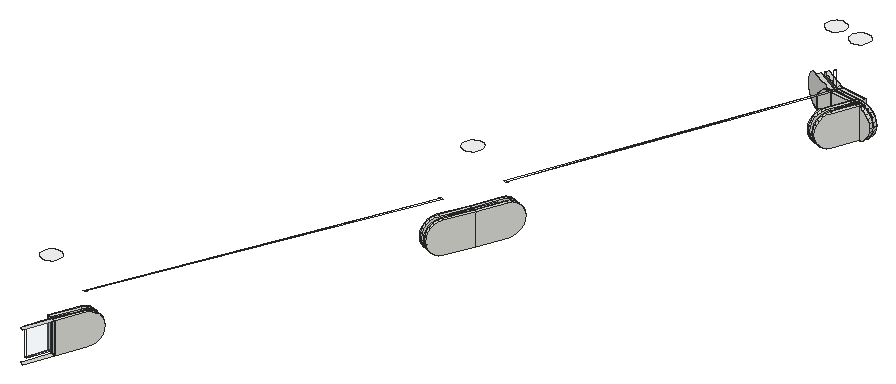
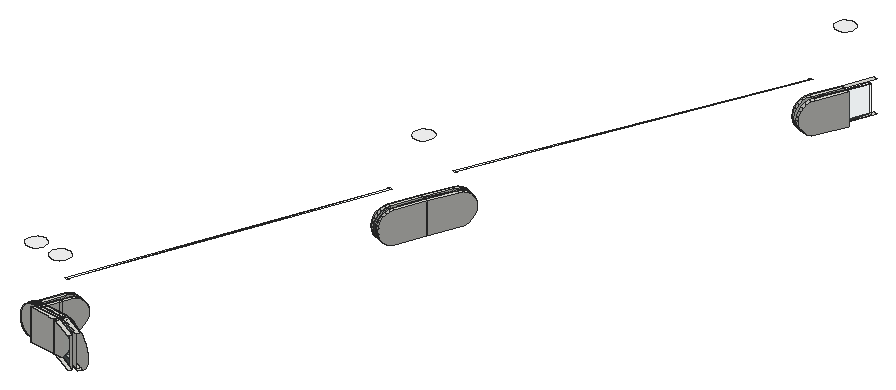
# SketchUp Ruby script. Lengths in inches.
U = 1.inch
M = Sketchup.active_model
def pt(a) = Geom::Point3d.new(a.map { |v| v * U })
def face(e, loops, mat)
  f = e.add_face(loops[0].map { |a| pt(a) })
  loops[1..].each { |l| e.add_face(l.map { |a| pt(a) }).erase! }
  f.material = f.back_material = mat if mat
  f
end
# faces: each face lists its corners as indices into pts; further lists are holes
def faces(e, pts, list, mat = nil) = list.each { |f| face(e, (f[0].is_a?(Array) ? f : [f]).map { |l| l.map { |i| pts[i] } }, mat) }
# xy, xz, yz: faces in a plane at the given z, y or x. An outline is a flat list of corners, or four numbers for a rectangle; further outlines are holes
def ring(l) = l.size == 4 ? [[l[0], l[1]], [l[2], l[1]], [l[2], l[3]], [l[0], l[3]]] : l.each_slice(2).to_a
def flat(e, list, mat, &to3) = list.each { |f| face(e, (f[0].is_a?(Array) ? f : [f]).map { |l| ring(l).map { |u, v| to3.(u, v) } }, mat) }
def xy(e, z, list, mat = nil) = flat(e, list, mat) { |x, y| [x, y, z] }
def xz(e, y, list, mat = nil) = flat(e, list, mat) { |x, z| [x, y, z] }
def yz(e, x, list, mat = nil) = flat(e, list, mat) { |y, z| [x, y, z] }
def lines(e, pts, list) = list.each { |a, b| e.add_line(pt(pts[a]), pt(pts[b])) }
# prism: a flat outline (further loops are holes) pulled along v
def prism(e, loops, v, mat = nil)
  f = face(e, loops, mat); d = Geom::Vector3d.new(v.map { |x| x * U })
  f.pushpull(f.normal.samedirection?(d) ? d.length : -d.length)
end
def box(e, o, s, mat = nil) = prism(e, [[o, [o[0] + s[0], o[1], o[2]], [o[0] + s[0], o[1] + s[1], o[2]], [o[0], o[1] + s[1], o[2]]]], [0, 0, s[2]], mat)
def at(x, y, z, deg = 0) = Geom::Transformation.translation(pt([x, y, z])) * Geom::Transformation.rotation(ORIGIN, Z_AXIS, deg.degrees)
def axes(o, x, y, z) = Geom::Transformation.new([*x, 0, *y, 0, *z, 0, *pt(o).to_a, 1])
def part(name) = M.definitions.add(name)
# library, detail: a bought-in or finely detailed component or shape, given as its bounding box
def library(name, o, s) = part(name).tap { |d| box(d.entities, o, s) }
def detail(e, o, s) = box(e.add_group.entities, o, s)
def put(e, d, t, mat = nil) = e.add_instance(d, t).tap { |i| i.material = mat if mat }
def group(e, t, mat = nil) = e.add_group.tap { |g| g.transformation = t; g.material = mat if mat }.entities
root = M.entities
M.materials.add("Glass_Safety_01").color = [204, 235, 244]
M.materials["Glass_Safety_01"].alpha = 0.1
M.materials.add("[Color_000]").color = [255, 255, 255]
xy(root,351.283,[[963.05,809.92,962.794,810.021,962.855,810.177,963.512,811.85,963.765,811.74],[963.765,811.74,963.512,811.85,963.513,811.853,963.77,811.753,963.767,811.746],[963.77,811.753,963.513,811.853,964.298,813.655,964.551,813.545],[963.332,811.929,963.079,812.039,963.865,813.843,964.118,813.733],[973.145,833.277,972.892,833.387,972.953,833.526,973.678,835.192,973.931,835.082],
  [972.711,833.465,972.459,833.576,973.241,835.37,973.496,835.268,972.772,833.605],[973.935,835.091,973.679,835.194,974.413,837.021,974.669,836.918],[973.496,835.268,973.241,835.37,973.245,835.38,973.497,835.27],[973.497,835.27,973.245,835.38,973.975,837.197,974.231,837.094],[982.068,855.317,981.812,855.42,981.873,855.571,982.412,856.912,982.491,856.9,982.519,857.095,982.531,857.173,982.539,857.227,982.546,857.247,982.802,857.144],
  [981.629,855.494,981.374,855.596,981.931,856.982,982.211,856.941,981.69,855.645],[982.491,856.9,982.412,856.912,982.487,857.1,982.519,857.095],[982.412,856.912,982.401,856.913,982.43,857.108,982.487,857.1],[982.401,856.913,982.211,856.941,982.287,857.129,982.43,857.108],[982.211,856.941,981.931,856.982,982.006,857.17,982.287,857.129],
  [981.931,856.982,980.543,857.184,980.572,857.379,982.006,857.17],[982.519,857.095,982.487,857.1,982.518,857.175,982.531,857.173],[982.487,857.1,982.43,857.108,982.441,857.186,982.518,857.175],[982.43,857.108,982.287,857.129,982.317,857.204,982.441,857.186],[982.287,857.129,982.006,857.17,982.037,857.245,982.317,857.204],
  [982.006,857.17,980.572,857.379,980.583,857.457,982.037,857.245],[982.531,857.173,982.518,857.175,982.539,857.227],[982.518,857.175,982.441,857.186,982.317,857.204,982.364,857.32,982.108,857.423,982.037,857.245,980.583,857.457,980.611,857.652,980.63,857.649,980.646,857.64,980.649,857.646,982.469,857.381,982.559,857.368,982.539,857.227],[980.543,857.184,980.453,857.197,980.474,857.338,980.545,857.462,980.583,857.457,980.572,857.379],[982.317,857.204,982.037,857.245,982.108,857.423,982.364,857.32],
  [980.412,857.229,978.702,858.205,978.839,858.444,980.548,857.469,980.545,857.462,980.493,857.47,980.474,857.338],[980.474,857.338,980.493,857.47,980.545,857.462],[982.469,857.381,980.649,857.646,980.782,857.879,980.721,857.914,982.509,857.653],[980.646,857.64,980.63,857.649,980.649,857.646],[980.649,857.646,980.63,857.649,980.528,857.707,980.561,857.9375,980.721,857.914,980.782,857.879],
  [980.63,857.649,980.611,857.652,980.521,857.665,980.528,857.707],[980.528,857.707,978.936,858.615,979.073,858.855,980.721,857.914,980.561,857.9375]])
xy(root,351.362,[[962.9375,810.388,962.754,810.46,963.33,811.925,963.422,811.889,963.512,811.85],[963.512,811.85,963.422,811.889,963.513,811.853,963.513,811.852],[963.513,811.853,963.422,811.889,963.332,811.929,963.96,813.372,964.141,813.294],[973.049,833.748,972.869,833.826,973.496,835.268,973.588,835.231,973.678,835.192],[973.679,835.194,973.588,835.231,973.497,835.27,974.084,836.729,974.267,836.655],
  [973.588,835.231,973.496,835.268,973.497,835.269,973.497,835.27],[981.959,855.785,981.776,855.859,982.317,857.204,982.441,857.186,982.455,857.283,982.546,857.247],[982.441,857.186,982.317,857.204,982.364,857.32,982.455,857.283],[982.317,857.204,982.141,857.23,982.17,857.424,982.469,857.381,982.455,857.283,982.364,857.32],[982.141,857.23,980.883,857.413,980.911,857.608,982.17,857.424],
  [980.883,857.413,980.583,857.457,980.597,857.554,980.646,857.64,980.63,857.649,980.911,857.608],[980.548,857.469,979.181,858.249,979.278,858.42,980.63,857.649,980.611,857.652,980.597,857.554],[980.597,857.554,980.611,857.652,980.63,857.649,980.646,857.64]],"Glass_Safety_01")
xy(root,353.33,[[962.9375,810.388,963.512,811.85,963.422,811.889,963.33,811.925,962.754,810.46],[963.512,811.85,963.513,811.852,963.513,811.853,963.422,811.889],[963.513,811.853,964.141,813.294,963.96,813.372,963.332,811.929,963.422,811.889],[973.049,833.748,973.678,835.192,973.588,835.231,973.496,835.268,972.869,833.826],[973.679,835.194,974.267,836.655,974.084,836.729,973.497,835.27,973.588,835.231],
  [973.588,835.231,973.497,835.27,973.497,835.269,973.496,835.268],[981.959,855.785,982.546,857.247,982.455,857.283,982.441,857.186,982.317,857.204,981.776,855.859],[982.441,857.186,982.455,857.283,982.364,857.32,982.317,857.204],[982.317,857.204,982.364,857.32,982.455,857.283,982.469,857.381,982.17,857.424,982.141,857.23],[982.141,857.23,982.17,857.424,980.911,857.608,980.883,857.413],
  [980.883,857.413,980.911,857.608,980.63,857.649,980.646,857.64,980.597,857.554,980.583,857.457],[980.548,857.469,980.597,857.554,980.611,857.652,980.63,857.649,979.278,858.42,979.181,858.249],[980.597,857.554,980.646,857.64,980.63,857.649,980.611,857.652]],"Glass_Safety_01")
xy(root,353.409,[[963.05,809.92,963.765,811.74,963.512,811.85,962.855,810.177,962.794,810.021],[963.765,811.74,963.767,811.746,963.77,811.753,963.513,811.853,963.512,811.85],[963.77,811.753,964.551,813.545,964.298,813.655,963.513,811.853],[963.332,811.929,964.118,813.733,963.865,813.843,963.079,812.039],[973.145,833.277,973.931,835.082,973.678,835.192,972.953,833.526,972.892,833.387],
  [972.711,833.465,972.772,833.605,973.496,835.268,973.241,835.37,972.459,833.576],[973.935,835.091,974.669,836.918,974.413,837.021,973.679,835.194],[973.496,835.268,973.497,835.27,973.245,835.38,973.241,835.37],[973.497,835.27,974.231,837.094,973.975,837.197,973.245,835.38],[982.068,855.317,982.802,857.144,982.546,857.247,982.539,857.227,982.531,857.173,982.519,857.095,982.491,856.9,982.412,856.912,981.873,855.571,981.812,855.42],
  [981.629,855.494,981.69,855.645,982.211,856.941,981.931,856.982,981.374,855.596],[982.491,856.9,982.519,857.095,982.487,857.1,982.412,856.912],[982.412,856.912,982.487,857.1,982.43,857.108,982.401,856.913],[982.401,856.913,982.43,857.108,982.287,857.129,982.211,856.941],[982.211,856.941,982.287,857.129,982.006,857.17,981.931,856.982],
  [981.931,856.982,982.006,857.17,980.572,857.379,980.543,857.184],[982.519,857.095,982.531,857.173,982.518,857.175,982.487,857.1],[982.487,857.1,982.518,857.175,982.441,857.186,982.43,857.108],[982.43,857.108,982.441,857.186,982.317,857.204,982.287,857.129],[982.287,857.129,982.317,857.204,982.037,857.245,982.006,857.17],
  [982.006,857.17,982.037,857.245,980.583,857.457,980.572,857.379],[982.531,857.173,982.539,857.227,982.518,857.175],[982.518,857.175,982.539,857.227,982.559,857.368,982.469,857.381,980.649,857.646,980.646,857.64,980.63,857.649,980.611,857.652,980.583,857.457,982.037,857.245,982.108,857.423,982.364,857.32,982.317,857.204,982.441,857.186],[980.543,857.184,980.572,857.379,980.583,857.457,980.545,857.462,980.474,857.338,980.453,857.197],[982.317,857.204,982.364,857.32,982.108,857.423,982.037,857.245],
  [980.412,857.229,980.474,857.338,980.493,857.47,980.545,857.462,980.548,857.469,978.839,858.444,978.702,858.205],[980.474,857.338,980.545,857.462,980.493,857.47],[982.469,857.381,982.509,857.653,980.721,857.914,980.782,857.879,980.649,857.646],[980.646,857.64,980.649,857.646,980.63,857.649],[980.649,857.646,980.782,857.879,980.721,857.914,980.561,857.9375,980.528,857.707,980.63,857.649],
  [980.63,857.649,980.528,857.707,980.521,857.665,980.611,857.652],[980.528,857.707,980.561,857.9375,980.721,857.914,979.073,858.855,978.936,858.615]])
xy(root,354.511,[[964.298,813.655,972.772,833.605,964.118,813.733],[964.298,813.655,972.953,833.526,972.772,833.605],[974.413,837.021,981.69,855.645,974.231,837.094],[974.413,837.021,981.873,855.571,981.69,855.645],[980.493,857.47,980.521,857.665,980.489,857.471],
  [980.489,857.471,980.521,857.665,980.517,857.665]],"Glass_Safety_01")
xy(root,357.267,[[963.467,811.261,963.628,811.294,963.775,811.368,963.898,811.477,963.988,811.614,964.04,811.77,964.05,811.934,964.017,812.096,963.943,812.243,963.834,812.366,963.697,812.456,963.541,812.508,963.377,812.518,963.216,812.485,963.069,812.411,962.946,812.302,962.855,812.165,962.803,812.008,962.793,811.844,962.827,811.683,962.9,811.536,963.009,811.413,963.147,811.323,963.303,811.271],[973.633,834.603,973.794,834.636,973.941,834.709,974.064,834.818,974.154,834.956,974.206,835.112,974.216,835.276,974.183,835.437,974.109,835.584,974,835.707,973.863,835.798,973.707,835.849,973.543,835.859,973.382,835.826,973.235,835.753,973.112,835.643,973.021,835.506,972.969,835.35,972.959,835.186,972.992,835.025,973.066,834.878,973.175,834.755,973.3125,834.664,973.469,834.612],[982.5,856.655,982.661,856.688,982.808,856.762,982.931,856.871,983.022,857.008,983.074,857.164,983.083,857.328,983.05,857.489,982.977,857.636,982.868,857.759,982.73,857.85,982.574,857.902,982.41,857.912,982.249,857.878,982.102,857.805,981.979,857.696,981.888,857.558,981.837,857.402,981.827,857.238,981.86,857.077,981.934,856.93,982.043,856.807,982.18,856.717,982.336,856.665],[980.642,856.926,980.803,856.959,980.95,857.033,981.073,857.142,981.164,857.279,981.216,857.435,981.225,857.599,981.192,857.76,981.119,857.907,981.01,858.03,980.872,858.121,980.716,858.173,980.552,858.183,980.391,858.15,980.244,858.076,980.121,857.967,980.03,857.829,979.979,857.673,979.969,857.509,980.002,857.348,980.075,857.201,980.185,857.078,980.322,856.988,980.478,856.936]],"[Color_000]")
xz(root,857.665,[[980.521,351.283,980.517,351.284,980.517,353.408,980.521,353.409],[980.517,353.408,980.517,354.511,980.521,354.511,980.521,353.409]],"Glass_Safety_01")
p = [[963.512,811.85,351.362],[963.512,811.85,351.283],[963.765,811.74,351.283],[963.765,811.74,353.409],[963.512,811.85,353.409],[963.512,811.85,353.33],
  [963.767,811.746,353.409],[963.767,811.746,351.283],[963.77,811.753,351.283],[963.77,811.753,353.409],[964.551,813.545,351.283],[964.661,813.797,351.319],
  [964.763,814.032,351.425],[964.851,814.234,351.594],[964.918,814.389,351.814],[964.961,814.486,352.071],[964.975,814.519,352.346],[964.961,814.486,352.621],
  [964.918,814.389,352.877],[964.851,814.234,353.098],[964.763,814.032,353.267],[964.661,813.797,353.373],[964.551,813.545,353.409],[963.513,811.853,351.283],
  [963.513,811.853,351.362],[963.513,811.853,353.33],[963.513,811.853,353.409],[963.33,811.925,351.362],[963.33,811.925,351.283],[963.074,812.026,351.283],
  [963.074,812.026,353.409],[963.33,811.925,353.409],[963.33,811.925,353.33],[963.332,811.929,351.283],[963.332,811.929,351.362],[963.332,811.929,353.33],
  [963.332,811.929,353.409],[963.079,812.039,353.409],[963.079,812.039,351.283],[964.118,813.733,351.283],[964.118,813.733,353.409],[963.96,813.372,353.33],
  [963.96,813.372,351.362],[964.298,813.655,353.409],[964.408,813.907,353.373],[964.51,814.142,353.267],[964.598,814.344,353.098],[964.666,814.499,352.877],
  [964.708,814.596,352.621],[964.723,814.629,352.346],[964.708,814.596,352.071],[964.666,814.499,351.814],[964.598,814.344,351.594],[964.51,814.142,351.425],
  [964.408,813.907,351.319],[964.298,813.655,351.283],[963.865,813.843,353.409],[963.975,814.096,353.373],[964.077,814.331,353.267],[964.165,814.533,353.098],
  [964.232,814.6875,352.877],[964.275,814.785,352.621],[964.289,814.818,352.346],[964.275,814.785,352.071],[964.232,814.6875,351.814],[964.165,814.533,351.594],
  [964.077,814.331,351.425],[963.975,814.096,351.319],[963.865,813.843,351.283],[964.227,813.986,351.319],[964.227,813.986,353.373],[964.33,814.221,353.267],
  [964.418,814.423,353.098],[964.485,814.577,352.877],[964.528,814.675,352.621],[964.542,814.708,352.346],[964.528,814.675,352.071],[964.485,814.577,351.814],
  [964.418,814.423,351.594],[964.33,814.221,351.425],[973.931,835.082,353.409],[973.145,833.277,353.409],[973.035,833.025,353.373],[972.932,832.79,353.267],
  [972.844,832.588,353.098],[972.777,832.433,352.877],[972.735,832.335,352.621],[972.72,832.302,352.346],[972.735,832.335,352.071],[972.777,832.433,351.814],
  [972.844,832.588,351.594],[972.932,832.79,351.425],[973.035,833.025,351.319],[973.145,833.277,351.283],[973.931,835.082,351.283],[972.892,833.387,353.409],
  [972.953,833.526,353.409],[972.953,833.526,351.283],[972.892,833.387,351.283],[972.782,833.135,351.319],[972.68,832.9,351.425],[972.592,832.698,351.594],
  [972.524,832.543,351.814],[972.482,832.446,352.071],[972.467,832.412,352.346],[972.482,832.446,352.621],[972.524,832.543,352.877],[972.592,832.698,353.098],
  [972.68,832.9,353.267],[972.782,833.135,353.373],[972.711,833.465,351.283],[972.772,833.605,351.283],[973.496,835.268,351.283],[973.496,835.268,351.362],
  [973.496,835.268,353.33],[973.496,835.268,353.409],[972.772,833.605,353.409],[972.711,833.465,353.409],[972.602,833.213,353.373],[972.499,832.978,353.267],
  [972.411,832.776,353.098],[972.344,832.621,352.877],[972.301,832.524,352.621],[972.287,832.491,352.346],[972.301,832.524,352.071],[972.344,832.621,351.814],
  [972.411,832.776,351.594],[972.499,832.978,351.425],[972.602,833.213,351.319],[972.459,833.576,353.409],[973.241,835.37,353.409],[973.241,835.37,351.283],
  [972.459,833.576,351.283],[972.349,833.323,351.319],[972.247,833.088,351.425],[972.159,832.886,351.594],[972.091,832.732,351.814],[972.049,832.634,352.071],
  [972.034,832.601,352.346],[972.049,832.634,352.621],[972.091,832.732,352.877],[972.159,832.886,353.098],[972.247,833.088,353.267],[972.349,833.323,353.373],
  [973.678,835.192,351.283],[973.678,835.192,353.409],[973.678,835.192,353.33],[973.049,833.748,353.33],[973.049,833.748,351.362],[973.678,835.192,351.362],
  [973.679,835.194,351.362],[973.679,835.194,351.283],[973.935,835.091,351.283],[973.935,835.091,353.409],[973.679,835.194,353.409],[973.679,835.194,353.33],
  [974.669,836.918,353.409],[974.669,836.918,351.283],[974.772,837.173,351.319],[974.867,837.411,351.425],[974.95,837.615,351.594],[975.013,837.772,351.814],
  [975.052,837.87,352.071],[975.066,837.904,352.346],[975.052,837.87,352.621],[975.013,837.772,352.877],[974.95,837.615,353.098],[974.867,837.411,353.267],
  [974.772,837.173,353.373],[974.413,837.021,353.409],[974.413,837.021,351.283],[974.267,836.655,351.362],[974.267,836.655,353.33],[973.497,835.27,351.362],
  [973.497,835.27,351.283],[973.245,835.38,351.283],[973.245,835.38,353.409],[973.497,835.27,353.409],[973.497,835.27,353.33],[974.231,837.094,351.283],
  [974.333,837.349,351.319],[974.429,837.587,351.425],[974.511,837.791,351.594],[974.574,837.948,351.814],[974.614,838.047,352.071],[974.627,838.08,352.346],
  [974.614,838.047,352.621],[974.574,837.948,352.877],[974.511,837.791,353.098],[974.429,837.587,353.267],[974.333,837.349,353.373],[974.231,837.094,353.409],
  [973.243,835.375,351.283],[973.243,835.375,353.409],[973.975,837.197,353.409],[974.078,837.452,353.373],[974.173,837.69,353.267],[974.256,837.894,353.098],
  [974.319,838.051,352.877],[974.358,838.149,352.621],[974.372,838.183,352.346],[974.358,838.149,352.071],[974.319,838.051,351.814],[974.256,837.894,351.594],
  [974.173,837.69,351.425],[974.078,837.452,351.319],[973.975,837.197,351.283],[974.516,837.276,351.319],[974.612,837.514,351.425],[974.694,837.718,351.594],
  [974.757,837.875,351.814],[974.797,837.973,352.071],[974.81,838.007,352.346],[974.797,837.973,352.621],[974.757,837.875,352.877],[974.694,837.718,353.098],
  [974.612,837.514,353.267],[974.516,837.276,353.373],[982.802,857.144,353.409],[982.068,855.317,353.409],[981.965,855.062,353.373],[981.869,854.824,353.267],
  [981.787,854.62,353.098],[981.724,854.463,352.877],[981.685,854.365,352.621],[981.671,854.331,352.346],[981.685,854.365,352.071],[981.724,854.463,351.814],
  [981.787,854.62,351.594],[981.869,854.824,351.425],[981.965,855.062,351.319],[982.068,855.317,351.283],[982.802,857.144,351.283],[981.812,855.42,353.409],
  [981.873,855.571,353.409],[981.873,855.571,351.283],[981.812,855.42,351.283],[981.709,855.165,351.319],[981.614,854.927,351.425],[981.532,854.723,351.594],
  [981.469,854.566,351.814],[981.429,854.468,352.071],[981.415,854.434,352.346],[981.429,854.468,352.621],[981.469,854.566,352.877],[981.532,854.723,353.098],
  [981.614,854.927,353.267],[981.709,855.165,353.373],[981.629,855.494,351.283],[981.69,855.645,351.283],[981.69,855.645,353.409],[981.629,855.494,353.409],
  [981.527,855.238,353.373],[981.431,855,353.267],[981.349,854.796,353.098],[981.286,854.639,352.877],[981.246,854.541,352.621],[981.233,854.507,352.346],
  [981.246,854.541,352.071],[981.286,854.639,351.814],[981.349,854.796,351.594],[981.431,855,351.425],[981.527,855.238,351.319],[982.037,857.245,353.409],
  [982.108,857.423,353.409],[982.108,857.423,351.283],[982.037,857.245,351.283],[982.006,857.17,351.283],[981.931,856.982,351.283],[981.374,855.596,351.283],
  [981.271,855.341,351.319],[981.175,855.103,351.425],[981.093,854.899,351.594],[981.03,854.742,351.814],[980.991,854.644,352.071],[980.977,854.61,352.346],
  [980.991,854.644,352.621],[981.03,854.742,352.877],[981.093,854.899,353.098],[981.175,855.103,353.267],[981.271,855.341,353.373],[981.374,855.596,353.409],
  [981.931,856.982,353.409],[982.006,857.17,353.409],[982.211,856.941,353.409],[982.211,856.941,351.283],[982.287,857.129,351.283],[982.317,857.204,351.283],
  [982.364,857.32,351.283],[982.364,857.32,351.362],[982.317,857.204,351.362],[981.776,855.859,351.362],[981.776,855.859,353.33],[982.317,857.204,353.33],
  [982.364,857.32,353.33],[982.364,857.32,353.409],[982.317,857.204,353.409],[982.287,857.129,353.409],[982.412,856.912,351.283],[982.412,856.912,353.409],
  [982.487,857.1,353.409],[982.518,857.175,353.409],[982.539,857.227,353.409],[982.546,857.247,353.409],[982.546,857.247,353.33],[981.959,855.785,353.33],
  [981.959,855.785,351.362],[982.546,857.247,351.362],[982.546,857.247,351.283],[982.539,857.227,351.283],[982.518,857.175,351.283],[982.487,857.1,351.283],
  [982.401,856.913,353.409],[982.401,856.913,351.283],[982.491,856.9,351.283],[982.763,856.86,351.319],[983.017,856.823,351.425],[983.235,856.792,351.594],
  [983.402,856.767,351.814],[983.507,856.752,352.071],[983.543,856.747,352.346],[983.507,856.752,352.621],[983.402,856.767,352.877],[983.235,856.792,353.098],
  [983.017,856.823,353.267],[982.763,856.86,353.373],[982.491,856.9,353.409],[982.792,857.055,351.319],[983.045,857.018,351.425],[980.543,857.184,353.409],
  [980.543,857.184,351.283],[980.572,857.379,353.409],[980.572,857.379,351.283],[982.43,857.108,351.283],[982.519,857.095,351.283],[983.263,856.986,351.594],
  [983.43,856.962,351.814],[983.535,856.947,352.071],[983.571,856.941,352.346],[983.535,856.947,352.621],[983.43,856.962,352.877],[983.263,856.986,353.098],
  [983.045,857.018,353.267],[982.792,857.055,353.373],[982.519,857.095,353.409],[982.43,857.108,353.409],[982.441,857.186,351.283],[982.441,857.186,351.362],
  [982.441,857.186,353.33],[982.441,857.186,353.409],[982.531,857.173,353.409],[982.803,857.133,353.373],[983.057,857.096,353.267],[983.275,857.064,353.098],
  [983.442,857.04,352.877],[983.547,857.025,352.621],[983.583,857.019,352.346],[983.547,857.025,352.071],[983.442,857.04,351.814],[983.275,857.064,351.594],
  [983.057,857.096,351.425],[982.803,857.133,351.319],[982.531,857.173,351.283],[982.559,857.368,351.283],[982.831,857.328,351.319],[983.085,857.291,351.425],
  [980.412,857.229,353.409],[978.702,858.205,353.409],[978.463,858.341,353.373],[978.24,858.468,353.267],[978.049,858.578,353.098],[977.902,858.661,352.877],
  [977.81,858.714,352.621],[977.779,858.732,352.346],[977.81,858.714,352.071],[977.902,858.661,351.814],[978.049,858.578,351.594],[978.24,858.468,351.425],
  [978.463,858.341,351.319],[978.702,858.205,351.283],[980.412,857.229,351.283],[980.453,857.197,351.283],[980.453,857.197,353.409],[980.181,857.237,353.373],
  [979.927,857.274,353.267],[979.709,857.306,353.098],[979.542,857.33,352.877],[979.437,857.345,352.621],[979.401,857.351,352.346],[979.437,857.345,352.071],
  [979.542,857.33,351.814],[979.709,857.306,351.594],[979.927,857.274,351.425],[980.181,857.237,351.319],[979.967,857.547,351.425],[980.221,857.51,351.319],
  [980.489,857.471,351.284],[980.493,857.47,351.283],[980.474,857.338,351.283],[980.548,857.469,351.283],[980.548,857.469,351.362],[980.548,857.469,353.33],
  [980.548,857.469,353.409],[980.545,857.462,353.409],[980.474,857.338,353.409],[980.545,857.462,351.283],[982.141,857.23,353.33],[982.141,857.23,351.362],
  [980.583,857.457,351.283],[980.583,857.457,351.362],[980.883,857.413,351.362],[980.883,857.413,353.33],[980.583,857.457,353.33],[980.583,857.457,353.409],
  [982.469,857.381,351.283],[982.469,857.381,351.362],[982.469,857.381,353.33],[982.469,857.381,353.409],[982.559,857.368,353.409],[982.831,857.328,353.373],
  [983.085,857.291,353.267],[983.303,857.259,353.098],[983.47,857.235,352.877],[983.575,857.219,352.621],[983.611,857.214,352.346],[983.575,857.219,352.071],
  [983.47,857.235,351.814],[983.303,857.259,351.594],[980.63,857.649,351.362],[980.911,857.608,351.362],[982.17,857.424,351.362],[980.649,857.646,351.283],
  [980.63,857.649,351.283],[980.611,857.652,351.283],[980.611,857.652,351.362],[982.509,857.653,351.283],[982.509,857.653,353.409],[978.839,858.444,351.283],
  [978.839,858.444,353.409],[979.181,858.249,353.33],[979.181,858.249,351.362],[980.221,857.51,353.373],[980.489,857.471,353.408],[979.749,857.578,351.594],
  [979.582,857.603,351.814],[979.477,857.618,352.071],[979.441,857.623,352.346],[979.477,857.618,352.621],[979.582,857.603,352.877],[979.749,857.578,353.098],
  [979.967,857.547,353.267],[980.493,857.47,353.409],[980.597,857.554,351.362],[980.528,857.707,353.409],[978.936,858.615,353.409],[978.936,858.615,351.283],
  [980.528,857.707,351.283],[980.646,857.64,351.283],[980.646,857.64,351.362],[979.278,858.42,351.362],[979.278,858.42,353.33],[980.63,857.649,353.33],
  [980.646,857.64,353.33],[980.646,857.64,353.409],[980.63,857.649,353.409],[980.782,857.879,351.283],[980.782,857.879,353.409],[980.649,857.646,353.409],
  [980.249,857.704,351.319],[980.517,857.665,351.284],[980.517,857.665,353.408],[980.249,857.704,353.373],[979.996,857.741,353.267],[979.778,857.773,353.098],
  [979.611,857.798,352.877],[979.505,857.813,352.621],[979.47,857.818,352.346],[979.505,857.813,352.071],[979.611,857.798,351.814],[979.778,857.773,351.594],
  [979.996,857.741,351.425],[980.721,857.914,353.409],[980.721,857.914,351.283],[980.561,857.9375,351.283],[980.289,857.977,351.319],[980.035,858.014,351.425],
  [979.817,858.046,351.594],[979.65,858.07,351.814],[979.545,858.086,352.071],[979.509,858.091,352.346],[979.545,858.086,352.621],[979.65,858.07,352.877],
  [979.817,858.046,353.098],[980.035,858.014,353.267],[980.289,857.977,353.373],[980.561,857.9375,353.409],[980.521,857.665,351.283],[980.611,857.652,353.409],
  [980.521,857.665,353.409],[980.611,857.652,353.33],[978.6,858.581,351.319],[962.9375,810.388,351.362],[962.9375,810.388,353.33],[962.754,810.46,353.33],
  [962.754,810.46,351.362],[963.422,811.889,353.33],[963.422,811.889,351.362],[963.513,811.852,351.362],[963.513,811.852,353.33],[964.141,813.294,353.33],
  [964.141,813.294,351.362],[972.869,833.826,353.33],[972.869,833.826,351.362],[973.588,835.231,351.362],[973.588,835.231,353.33],[973.497,835.269,353.33],
  [973.497,835.269,351.362],[974.084,836.729,351.362],[974.084,836.729,353.33],[982.17,857.424,353.33],[982.455,857.283,351.362],[982.455,857.283,353.33],
  [980.911,857.608,353.33],[980.597,857.554,353.33],[980.489,857.471,354.511],[980.493,857.47,354.511]]
faces(root,p,[[0,1,2,3,4,5],[6,3,2,7,8,9],[6,3,2,7,8,10,11,12,13,14,15,16,17,18,19,20,21,22,9],[23,24,25,26,9,8],[27,28,29,30,31,32],[33,34,35,36,37,38],[33,39,40,36,35,41,42,34],[23,1,0,5,4,26,25,24],
  [4,26,43,44,45,46,47,48,49,50,51,52,53,54,55,23,1,0,5],[37,56,57,58,59,60,61,62,63,64,65,66,67,68,38],[55,54,11,10],[69,39,68,67],[54,53,12,11],[79,69,67,66],[80,81,82,83,84,85,86,87,88,89,90,91,92,93,94],[95,96,97,98,99,100,101,102,103,104,105,106,107,108,109],
  [110,111,112,113,114,115,116,117,118,119,120,121,122,123,124,125,126,127,128],[129,130,131,132,133,134,135,136,137,138,139,140,141,142,143],[100,99,92,91],[128,127,134,133],[99,98,93,92],[110,128,133,132],[144,97,96,145,146,147,148,149],[144,149,146,145,80,94],
  [150,151,152,153,154,155],[156,153,152,157,158,159,160,161,162,163,164,165,166,167,168],[154,169,170,151,150,171,172,155],[112,113,114,115,130,131],[173,174,175,176,177,178],[177,115,114,113,112,174,173,178],[177,115,114,113,112,174,179,180,181,182,183,184,185,186,187,188,189,190,191],[192,131,130,193,176,175],
  [130,193,176,194,195,196,197,198,199,200,201,202,203,204,205,206,175,192,131],[170,207,158,157],[180,179,206,205],[207,208,159,158],[181,180,205,204],[218,219,220,221,222,223,224,225,226,227,228,229,230,231,232],[233,234,235,236,237,238,239,240,241,242,243,244,245,246,247],[248,249,250,251,252,253,254,255,256,257,258,259,260,261,262],
  [263,264,265,266,267,268,269,270,271,272,273,274,275,276,277,278,279,280,281,282,283],[238,237,230,229],[262,261,271,270],[237,236,231,230],[248,262,270,269],[284,250,249,285,286,287,288,289,290,291,292,293,294,295,296,297],[298,235,234,299,300,301,302,303,304,305,306,307,308,309,310,311],[299,312,313,298,314,315,316,317,318,319,320,321,322,323,324,325,326],
  [315,327,328,316],[285,313,312,284,282,329,330,268],[283,331,332,267,286,333,311,334,327,328,335,336,337,338,339,340,341,342,343,344,300,345,297],[346,347,348,349,345,312,313,333],[314,334,327,315],[310,346,347,348,349,301,350,351,352,353,354,355,356,357,358,359,360,361,362],[360,328,327,361],[361,327,334,362],
  [308,307,304,303,218,232],[363,364,361,362,309],[364,365,360,361],[366,367,368,369,370,371,372,373,374,375,376,377,378,379,380],[381,330,329,382,383,384,385,386,387,388,389,390,391,392,393],[394,395,393,392],[395,396,397,398,381,393],[399,400,401,402,403,404,366,380,398,405],
  [331,329,330,332],[296,349,348,293,406,407,290,347,346,287,266,408,409,410,411,412,413,263],[363,414,415,416,417,418,419,420,421,422,423,424,425,426,427,365,364],[289,288,265,264,295,294],[408,409,412,413,331,332],[428,429,430,415,414,431,432,433,434],[415,414,435,436,417,416],[399,437,438,402,401,439,440,400],
  [441,442,396,395,394,443,444,445,446,447,448,449,450],[403,413,412,409,408,405,397,451],[434,452,409,408,433],[453,454,455,456,432,457,458,428,459,460,461,462,463,464],[458,457,431,465,466,467,463,462],[468,469,470,471,472,473,474,475,476,477,478,479,480],[481,436,435,482,483,484,485,486,487,488,489,490,491,492,493,494,495],[468,480,485,484],
  [469,468,484,483,456,496],[497,498,496,433,434,499],[500,437,379,378],[53,52,13,12],[78,79,66,65],[101,100,91,90],[127,126,135,134],[208,209,160,159],
  [182,181,204,203],[239,238,229,228],[261,260,272,271],[316,328,335,317],[359,335,328,360],[365,427,359,360],[443,394,392,391],[409,412,411,410],
  [523,412,409,452],[480,479,486,485],[52,51,14,13],[77,78,65,64],[102,101,90,89],[126,125,136,135],[209,210,161,160],[183,182,203,202],
  [240,239,228,227],[260,259,273,272],[317,335,336,318],[358,336,335,359],[427,426,358,359],[444,443,391,390],[479,478,487,486],[51,50,15,14],
  [76,77,64,63],[103,102,89,88],[125,124,137,136],[210,211,162,161],[184,183,202,201],[241,240,227,226],[259,258,274,273],[318,336,337,319],
  [357,337,336,358],[426,425,357,358],[445,444,390,389],[478,477,488,487],[50,49,16,15],[75,76,63,62],[104,103,88,87],[124,123,138,137],
  [211,212,163,162],[185,184,201,200],[242,241,226,225],[258,257,275,274],[319,337,338,320],[356,338,337,357],[425,424,356,357],[446,445,389,388],
  [477,476,489,488],[49,48,17,16],[74,75,62,61],[105,104,87,86],[123,122,139,138],[212,213,164,163],[186,185,200,199],[243,242,225,224],
  [257,256,276,275],[320,338,339,321],[355,339,338,356],[424,423,355,356],[447,446,388,387],[476,475,490,489],[48,47,18,17],[73,74,61,60],
  [106,105,86,85],[122,121,140,139],[213,214,165,164],[187,186,199,198],[244,243,224,223],[256,255,277,276],[321,339,340,322],[354,340,339,355],
  [423,422,354,355],[448,447,387,386],[475,474,491,490],[47,46,19,18],[72,73,60,59],[107,106,85,84],[121,120,141,140],[214,215,166,165],
  [188,187,198,197],[245,244,223,222],[255,254,278,277],[322,340,341,323],[353,341,340,354],[422,421,353,354],[449,448,386,385],[474,473,492,491],
  [46,45,20,19],[71,72,59,58],[108,107,84,83],[120,119,142,141],[215,216,167,166],[189,188,197,196],[246,245,222,221],[254,253,279,278],
  [323,341,342,324],[352,342,341,353],[421,420,352,353],[450,449,385,384],[473,472,493,492],[45,44,21,20],[70,71,58,57],[109,108,83,82],
  [119,118,143,142],[216,217,168,167],[190,189,196,195],[247,246,221,220],[253,252,280,279],[324,342,343,325],[351,343,342,352],[420,419,351,352],
  [441,450,384,383],[416,519,522,461,499,497,464,467,417],[497,413,412,523,499],[472,471,494,493],[44,43,22,21],[40,70,57,56],[95,109,82,81],[118,117,129,143],
  [217,169,156,168],[191,190,195,194],[233,247,220,219],[252,251,281,280],[343,325,326,344],[350,302,418,419,351,343,344],[451,442,441,383,382,404],[470,498,453,495,494,471]])
faces(root,p,[[39,40,70,71,72,73,74,75,76,77,78,79,69],[43,55,54,53,52,51,50,49,48,47,46,45,44],[169,170,207,208,209,210,211,212,213,214,215,216,217],[179,191,190,189,188,187,186,185,184,183,182,181,180],[442,396,397,451],[501,0,5,502],[32,503,504,27],[32,505,506,27],
  [506,505,35,34],[41,35,34,42],[505,506,0,5],[24,506,505,25],[507,24,25,508,5,0],[509,25,24,510],[41,509,510,42],[511,512,148,147],
  [147,146,149,148],[511,114,113,512],[513,514,114,113],[178,514,513,173],[149,513,514,146],[514,513,150,155],[155,172,171,150],[515,178,173,516,113,114],
  [517,173,178,518],[171,517,518,172],[292,291,306,305],[305,304,307,306],[294,293,292,291,290,289],[406,411,410,407],[406,293,348,347,290,407],[406,407,430,519],
  [520,521,348,347],[307,520,521,304],[294,521,520,289],[521,520,415,416],[429,410,411,522],[522,519,430,429],[415,430,519,416],[439,401,400,440],
  [452,523,401,400],[462,461,460,459,428,458],[523,452,458,462],[452,434,499,523],[499,461,522,429,428,434],[439,460,459,440],[524,442,451,525]],"Glass_Safety_01")
